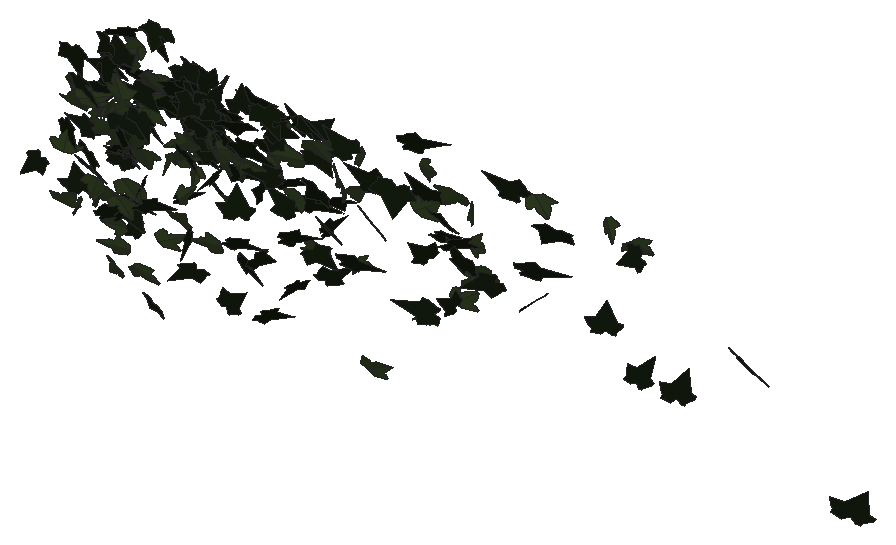
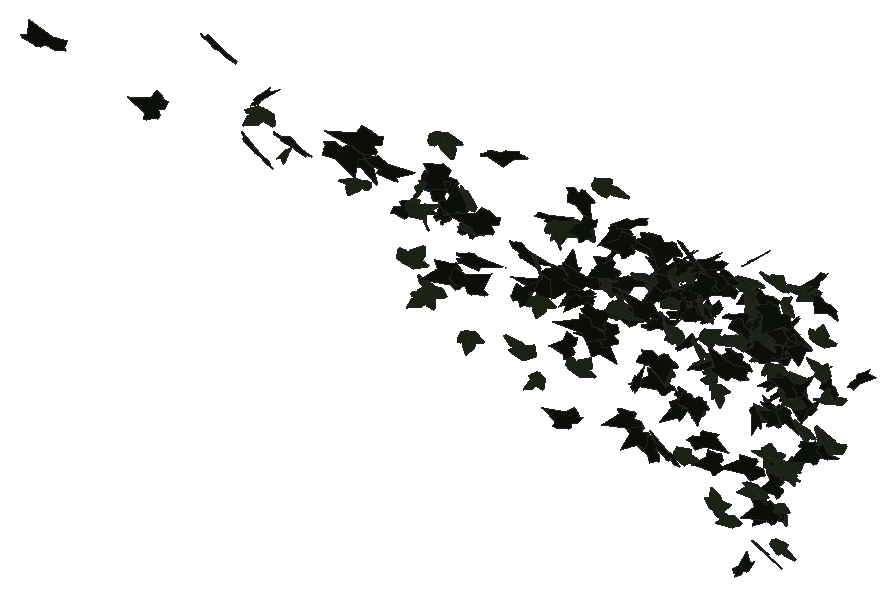
# SketchUp Ruby script. Lengths in millimetres.
U = 1.mm
M = Sketchup.active_model
def pt(a) = Geom::Point3d.new(a.map { |v| v * U })
def face(e, loops, mat)
  f = e.add_face(loops[0].map { |a| pt(a) })
  loops[1..].each { |l| e.add_face(l.map { |a| pt(a) }).erase! }
  f.material = f.back_material = mat if mat
  f
end
# faces: each face lists its corners as indices into pts; further lists are holes
def faces(e, pts, list, mat = nil) = list.each { |f| face(e, (f[0].is_a?(Array) ? f : [f]).map { |l| l.map { |i| pts[i] } }, mat) }
# xy, xz, yz: faces in a plane at the given z, y or x. An outline is a flat list of corners, or four numbers for a rectangle; further outlines are holes
def ring(l) = l.size == 4 ? [[l[0], l[1]], [l[2], l[1]], [l[2], l[3]], [l[0], l[3]]] : l.each_slice(2).to_a
def flat(e, list, mat, &to3) = list.each { |f| face(e, (f[0].is_a?(Array) ? f : [f]).map { |l| ring(l).map { |u, v| to3.(u, v) } }, mat) }
def xy(e, z, list, mat = nil) = flat(e, list, mat) { |x, y| [x, y, z] }
def xz(e, y, list, mat = nil) = flat(e, list, mat) { |x, z| [x, y, z] }
def yz(e, x, list, mat = nil) = flat(e, list, mat) { |y, z| [x, y, z] }
def lines(e, pts, list) = list.each { |a, b| e.add_line(pt(pts[a]), pt(pts[b])) }
# prism: a flat outline (further loops are holes) pulled along v
def prism(e, loops, v, mat = nil)
  f = face(e, loops, mat); d = Geom::Vector3d.new(v.map { |x| x * U })
  f.pushpull(f.normal.samedirection?(d) ? d.length : -d.length)
end
def box(e, o, s, mat = nil) = prism(e, [[o, [o[0] + s[0], o[1], o[2]], [o[0] + s[0], o[1] + s[1], o[2]], [o[0], o[1] + s[1], o[2]]]], [0, 0, s[2]], mat)
def at(x, y, z, deg = 0) = Geom::Transformation.translation(pt([x, y, z])) * Geom::Transformation.rotation(ORIGIN, Z_AXIS, deg.degrees)
def axes(o, x, y, z) = Geom::Transformation.new([*x, 0, *y, 0, *z, 0, *pt(o).to_a, 1])
def part(name) = M.definitions.add(name)
# library, detail: a bought-in or finely detailed component or shape, given as its bounding box
def library(name, o, s) = part(name).tap { |d| box(d.entities, o, s) }
def detail(e, o, s) = box(e.add_group.entities, o, s)
def put(e, d, t, mat = nil) = e.add_instance(d, t).tap { |i| i.material = mat if mat }
def group(e, t, mat = nil) = e.add_group.tap { |g| g.transformation = t; g.material = mat if mat }.entities
root = M.entities
M.materials.add("efeu1").color = [18, 25, 13]
M.materials.add("efeu2").color = [43, 57, 29]
c1 = part("ivyleaf_10")
p = [[0,12.8,-0.8],[-1.5,51.3,-10.9],[-4.9,51,-11.6],[-13.6,26.5,-7.3],[-13.2,15.9,-4.6],[-21.1,19.3,-7.2],
  [-29.5,16.3,-8.3],[-29.2,8.3,-6.2],[-19.7,-9.8,0.5],[-7.6,-13,4],[1,-12.2,5.8],[-0.4,51.1,-11.1],
  [-1.5,51.1,-10.9],[1,-12.4,5.9],[16.9,-12.4,3.5],[35.1,9.1,-5.1],[35,12.9,-6.1],[20.5,16.4,-4.9],
  [15.8,15,-3.8],[15.3,27.6,-7.1],[12.8,31.3,-7.8]]
faces(c1.entities,p,[[0,1,2,3,4,5,6,7,8,9,10],[11,12,0,13,14,15,16,17,18,19,20]],"efeu2")
c2 = part("ivyleaf_9")
p = [[39.1,54.8,31.7],[34.5,51.8,30.2],[-5.3,25.2,17.3],[-17.9,28.3,20.9],[-21.6,21.7,17],[-20.2,4.3,5.3],
  [-22.9,-0.3,2.5],[-17.1,-4,-0.6],[-2,-2.1,-1.2],[-0.7,-15.4,-10.1],[16.6,-22.3,-16.7],[21.1,-15.1,-12.5],
  [32.7,-10.7,-11],[46.1,-1.8,-6.6],[30.8,11.2,3.8]]
faces(c2.entities,p,[[0,1,2,3,4,5,6,7,8,9,10,11,12,13,14]],"efeu1")
put(root,c1,axes([5064.2,937.7,790.6],[0.67304,-0.23395,-0.96533],[-1.59231,0.48213,-0.42334],[1.0189,0.908,-0.02393]))
put(root,c1,axes([5001.8,756.4,1400.4],[-0.8248,0.04636,1.15791],[2.09058,-0.37742,0.42623],[0.70265,1.17734,0.09105]))
put(root,c2,axes([5054.6,918.4,1310.9],[-0.906,0.80347,-0.50065],[0.44749,-0.44248,-0.93368],[-1.74528,-0.53054,0.0205]))
put(root,c2,axes([5052.5,851.7,1350.8],[-0.03456,-0.01498,1.10733],[-1.36507,-0.84365,-0.02318],[1.60586,-0.71747,0.00413]))
put(root,c2,axes([5008.5,928.6,1425.8],[0.54035,-0.11605,-1.00857],[1.93217,0.03577,0.28167],[0.00611,-1.04716,0.12139]))
put(root,c2,axes([5023.9,778.4,1101],[1.95729,-0.44574,-0.06664],[-0.11819,0.02431,-1.12086],[0.84959,1.03029,-0.00239]))
put(root,c2,axes([5063,493,1250],[0.21616,-0.29781,-1.14485],[0.79529,-1.06587,0.31872],[-2.10625,-0.43302,0.00285]))
put(root,c2,axes([5081.5,705.2,1045.3],[-2.0987,-0.07093,0.2202],[0.4185,0.01182,1.105],[-0.13678,1.12443,0.00227]))
put(root,c1,axes([5057,640.6,1228.6],[1.69953,0.65213,-0.2656],[0.37803,0.17823,1.10545],[1.2857,-0.91444,0.02605]))
put(root,c2,axes([5045.2,662.6,1306.6],[-0.5613,0.05695,-1.17254],[2.19376,-0.21497,-0.30037],[-0.42323,-1.1898,-0.00186]))
put(root,c1,axes([5097.5,781.5,1320.9],[-0.42723,0.35407,1.05328],[-1.33204,0.78957,-0.41458],[-1.64262,-0.73237,0.06225]))
put(root,c1,axes([5069.2,624.9,1028.7],[-1.82637,-0.24048,0.45997],[0.87286,0.05985,0.98812],[-0.46254,1.06249,0.04845]))
put(root,c2,axes([5117.9,974.4,786.1],[-1.73472,0.56442,0.00038],[-0.00075,0.00009,-1.07208],[-1.0742,-0.91148,0.00014]))
put(root,c1,axes([5058.5,831,1298.2],[1.2924,-0.13297,-0.79694],[1.50662,-0.09878,0.69102],[-0.30766,-1.04235,0.03618]))
put(root,c2,axes([5078,657.6,1613.5],[-1.19341,-0.08927,-0.99726],[1.8737,0.15932,-0.6333],[0.34704,-1.16719,-0.01017]))
put(root,c1,axes([5100,775,1326.7],[0.10477,-1.00057,0.68235],[0.29766,-0.67147,-0.99722],[2.28566,0.13331,0.09859]))
put(root,c2,axes([5111.7,765.2,1278.7],[1.37307,0.31331,-0.76378],[-1.39675,-0.2211,-0.78392],[-0.71951,1.02712,0.06424]))
put(root,c2,axes([5105.9,820.3,1575.4],[-0.48565,-0.52996,0.88702],[-0.42571,-0.86368,-0.58036],[1.91991,-0.32557,0.09569]))
put(root,c2,axes([5130.5,687.2,1309.7],[-0.15478,-1.06398,-0.14432],[-0.02081,-0.14391,1.06708],[-2.04341,0.08206,0.00006]))
put(root,c1,axes([5140.4,794.6,1008.8],[-1.75315,0.04978,0.59176],[-1.12423,0.03547,-0.9225],[-0.11618,-1.09429,-0.00298]))
put(root,c1,axes([5132.4,618.4,1433.7],[-2.04621,0.21259,-0.09072],[-0.17772,-0.0047,1.09573],[0.40241,1.07895,0.02264]))
put(root,c2,axes([5116.7,781.6,1517],[0.72979,-0.5039,-1.08095],[-1.09473,0.91652,-0.6313],[1.98838,0.68955,0.04917]))
put(root,c2,axes([5092,932,909.9],[1.91135,0.05327,0.3186],[0.60672,0.00457,-1.00562],[-0.09927,1.0536,-0.01175]))
put(root,c2,axes([5103.9,712.7,1194.3],[0.13051,-0.86871,0.80221],[0.20025,-0.79588,-0.87086],[2.24152,0.12168,0.03109]))
put(root,c1,axes([5122.8,726.4,1012.3],[0.10372,-0.04255,-1.07115],[0.4224,1.04975,-0.03041],[1.99602,-0.21994,0.0621]))
put(root,c2,axes([5111.8,913.5,888.4],[-0.38965,-0.75246,-0.7988],[0.41389,0.76864,-0.7798],[2.04714,-0.29862,0.00562]))
put(root,c1,axes([5127.2,893.1,1101.8],[1.77653,0.55515,-0.12163],[0.16948,0.08812,1.08564],[1.06827,-0.9372,0.03003]))
put(root,c2,axes([5180.4,747.7,1527.9],[-0.73932,0.05518,-1.16046],[-2.21107,-0.01654,0.38811],[0.00344,1.22364,0.05758]))
put(root,c2,axes([5161.2,830.1,1519],[-2.17248,-0.10172,0.28438],[0.55274,-0.06455,1.14267],[-0.15776,1.17461,0.08742]))
put(root,c2,axes([5133.8,837.4,1630.3],[1.55878,0.87426,0.24465],[0.3207,0.17738,-1.19797],[-1.69779,0.83619,-0.00167]))
put(root,c1,axes([5152.2,602.8,1056.6],[0.49358,-1.13684,-0.16233],[-0.06031,0.15927,-1.16603],[2.18474,0.26123,0.00448]))
put(root,c2,axes([5161.3,722.3,1467.4],[1.32035,0.55576,-0.65751],[-0.96639,-0.41777,-0.88888],[-1.32317,0.8597,-0.0069]))
put(root,c1,axes([5185.8,723.3,1313.6],[-1.48603,-0.29671,0.77164],[-1.37717,-0.26803,-0.83527],[0.76094,-1.06454,-0.00477]))
put(root,c1,axes([5162.7,921.7,971.3],[1.56175,-0.62751,-0.26292],[-0.39992,0.15804,-1.03302],[1.23157,0.84707,-0.00204]))
put(root,c1,axes([5183.1,888.3,1555.9],[1.2385,-0.37421,-0.7487],[-1.25888,0.35123,-0.75045],[0.97616,0.92772,-0.01788]))
put(root,c1,axes([5155,684,1108.5],[1.9985,-0.54064,0.06378],[0.12765,-0.00903,-1.18086],[1.02818,1.05197,0.02264]))
put(root,c2,axes([5153.3,730.5,959],[0.20424,0.01435,1.07001],[1.70735,0.58507,-0.09782],[-1.11033,0.9023,0.0464]))
put(root,c2,axes([5167.5,798.2,924.4],[0.47641,0.37607,1.00371],[1.01539,0.85024,-0.45163],[-1.76927,0.58922,0.01108]))
put(root,c2,axes([5156.9,858.1,1469],[2.26962,-0.08387,-0.27225],[0.51652,-0.02173,1.19547],[-0.16481,-1.22302,-0.00257]))
put(root,c2,axes([5212.3,745.3,1430.6],[0.28079,-0.37544,1.02948],[-0.47608,0.9998,0.40047],[-2.03047,-0.28634,0.04847]))
put(root,c2,axes([5162.2,809.7,1197.8],[0.88049,-0.83971,0.54607],[0.55749,-0.46178,-0.95827],[1.823,0.54679,0.0293]))
put(root,c1,axes([5224.7,713.5,782.7],[-1.3865,0.38914,0.66141],[-1.12057,0.30146,-0.82588],[-0.9367,-0.93665,0.00898]))
put(root,c2,axes([5183.1,787.1,1326.2],[1.00325,-1.01866,0.01643],[0.01432,-0.01461,-1.14698],[1.93892,0.52719,-0.00003]))
put(root,c2,axes([5221.8,761,1240.2],[-0.60975,-0.56043,0.90184],[-0.88478,-0.77287,-0.64544],[1.8168,-0.56447,-0.01166]))
put(root,c2,axes([5213,748.8,1171.1],[-1.32421,0.67658,0.54301],[0.74321,-0.37732,0.9705],[1.47437,0.79787,-0.0015]))
put(root,c1,axes([5196.8,768.2,1005.9],[1.7398,0.19985,0.59739],[1.08677,0.18164,-0.93457],[-0.50621,1.07682,0.04678]))
put(root,c2,axes([5205.7,532.3,1596.1],[1.06998,-1.14469,-0.00344],[-0.00202,0.00331,-1.2753],[2.17858,0.5622,0.0005]))
put(root,c1,axes([5278.6,685.5,888.5],[0.01372,0.0139,1.08365],[-1.86185,-0.46623,0.01249],[0.88755,-0.97825,0.00945]))
put(root,c2,axes([5246.3,929.9,1627.8],[-1.21428,-0.87666,-0.02225],[0.0246,0.01811,-1.08425],[1.66881,-0.63815,-0.0002]))
put(root,c2,axes([5220.4,927.8,1594.9],[-0.4898,0.01277,-1.04929],[1.99688,-0.01471,-0.25752],[-0.03298,-1.08029,-0.0089]))
put(root,c1,axes([5269.3,717.8,1430.6],[1.30739,-0.61217,-0.63555],[-0.92869,0.40754,-0.91998],[1.3993,0.84245,-0.01677]))
put(root,c1,axes([5255.3,773.7,1553.5],[1.19116,-0.96913,0.5274],[-0.53739,0.44547,1.15365],[-2.02995,-0.68661,0.00407]))
put(root,c1,axes([5267,699.2,1308.1],[-1.13795,-0.9866,-0.20442],[0.22553,0.1672,-1.15354],[1.90426,-0.60937,0.01446]))
put(root,c1,axes([5237.4,526.7,1535.6],[0.89648,0.08984,-1.13989],[1.98945,0.46578,0.46867],[0.88192,-1.14205,0.10147]))
put(root,c2,axes([5250.3,829.5,988.4],[0.23583,0.43926,-1.00569],[0.47277,0.97459,0.45628],[2.03443,-0.2774,0.01055]))
put(root,c2,axes([5266.6,865.7,589],[1.21104,-0.642,-0.57517],[0.76326,-0.41233,0.9039],[-1.45212,-0.75214,-0.00458]))
put(root,c1,axes([5266,749.5,1384.8],[0.91172,0.46185,-0.89118],[1.22397,0.61694,0.66542],[1.46673,-0.80192,-0.00133]))
put(root,c2,axes([5283.3,805.8,1455.6],[0.45462,-0.51465,-1.0461],[1.05781,-0.88839,0.56399],[-1.95045,-0.60177,0.06204]))
put(root,c1,axes([5263.3,931.4,806.5],[1.31726,-0.04297,-0.81937],[1.56122,0.01368,0.69221],[-0.03286,-1.07249,0.04165]))
put(root,c1,axes([5298.1,598.8,1501.6],[0.50739,-0.99216,0.69498],[0.30977,-0.67582,-1.02724],[2.28454,0.312,-0.01506]))
put(root,c1,axes([5267.6,709.7,1124.4],[1.63569,0.05689,0.79181],[1.48973,0.13373,-0.85922],[-0.25177,1.16091,0.06018]))
put(root,c1,axes([5309.8,859.8,1485.3],[1.75949,0.48477,-0.38729],[-0.64796,-0.18468,-1.04387],[-0.98726,0.98517,-0.00511]))
put(root,c1,axes([5299.7,972.6,876.2],[-1.89439,0.16535,0.41323],[0.7465,-0.15257,1.00585],[0.40035,1.06688,0.0798]))
put(root,c2,axes([5326.2,721.5,1126.8],[-0.27138,0.12416,-1.22895],[-1.6277,0.88268,0.18841],[1.69618,0.86691,-0.01583]))
put(root,c1,axes([5275.4,770.5,1457.4],[0.62981,0.06052,-1.1124],[2.07001,0.23357,0.33627],[0.45883,-1.13683,0.00987]))
put(root,c2,axes([5280,866.3,1409.3],[-0.02432,0.0045,-1.1103],[1.94482,0.43433,-0.01],[0.82648,-1.02191,-0.00914]))
put(root,c2,axes([5293.9,668.2,1416.7],[-0.45715,-0.7174,-0.98343],[1.00062,0.84293,-0.74333],[2.08951,-0.56061,0.14081]))
put(root,c2,axes([5327.4,693.2,1331.7],[-0.86682,-0.7442,0.79182],[-0.69155,-0.70483,-0.87145],[1.94906,-0.58106,0.04295]))
put(root,c2,axes([5302.6,888.1,1354],[-0.92723,0.00001,1.14439],[1.86586,-0.64159,0.41738],[1.1235,1.06553,0.2513]))
put(root,c2,axes([5305.6,611,1324.6],[2.07086,0.26212,0.32005],[0.59143,0.0766,-1.11922],[-0.51973,1.1316,0.00162]))
put(root,c1,axes([5347.5,587.9,1564.7],[2.0483,-0.08575,0.44382],[-0.8361,0.07148,1.07913],[-0.20259,-1.16196,0.03363]))
put(root,c1,axes([5346.6,737.3,1573.4],[0.14783,-0.94291,0.60554],[0.18512,-0.59903,-0.94525],[2.12469,0.1178,0.04023]))
put(root,c1,axes([5323.8,711.2,810.7],[-1.24159,0.11669,-0.86899],[1.62988,-0.1475,-0.66272],[-0.35789,-1.07656,-0.00339]))
put(root,c2,axes([5340.9,915,1004.8],[0.66207,0.35599,0.95871],[1.35601,0.64209,-0.49695],[-1.39626,0.79238,-0.02802]))
put(root,c2,axes([5343.7,664.6,1554.9],[-0.6362,-0.44901,-1.13368],[1.50584,0.81456,-0.55592],[1.76578,-0.85642,0.06562]))
put(root,c2,axes([5345.1,582.9,1408.3],[0.24415,-0.08477,-1.23247],[2.26263,-0.3284,0.14633],[-0.63921,-1.19482,0.04722]))
put(root,c2,axes([5354,677.8,1454.4],[1.34868,-1.15375,-0.04659],[-0.02908,0.04529,-1.35395],[2.1974,0.70872,0.01068]))
put(root,c1,axes([5401.3,665,1473.9],[-0.03939,-1.07947,0.24208],[-0.02383,-0.24187,-1.07964],[2.10533,-0.02294,-0.00769]))
put(root,c1,axes([5402,840.1,1239],[-0.3553,-1.12325,-0.10035],[0.04219,0.09804,-1.13865],[2.14588,-0.18791,0.00577]))
put(root,c1,axes([5379.4,698,1587],[-0.61611,0.31033,-1.05872],[1.55034,-0.67688,-0.44749],[-1.41609,-0.87608,-0.02929]))
put(root,c1,axes([5412,572.4,1379.2],[-0.54332,-1.16466,-0.34594],[-0.15871,-0.33574,1.19914],[-2.30684,0.29741,-0.00102]))
put(root,c2,axes([5447,911.9,1216.2],[1.34732,0.21976,-0.8054],[-1.5276,-0.11126,-0.73587],[-0.43699,1.06651,0.08919]))
put(root,c1,axes([5447.4,875.8,1167.9],[0.26883,0.94566,-0.59477],[-0.21192,-0.5846,-0.95594],[-2.11557,0.17872,0.02018]))
put(root,c1,axes([5454.1,571.9,1373.5],[-2.17132,-0.33532,-0.23766],[0.4487,0.04044,-1.18883],[0.64072,-1.16467,0.02715]))
put(root,c2,axes([5478.9,855.5,1305.6],[-1.22545,-0.92695,0.25572],[0.27658,0.21041,1.12864],[-1.80905,0.66008,-0.00067]))
put(root,c1,axes([5455.8,720.6,1280.7],[0.22851,-0.39198,1.14556],[0.84926,-1.05582,-0.40804],[2.14213,0.4604,0.03957]))
put(root,c1,axes([5475.9,582.9,1530.2],[2.08777,0.24304,-0.16363],[-0.30359,-0.03646,-1.12358],[-0.46773,1.10852,-0.00108]))
put(root,c2,axes([5450,822.6,1618.8],[1.73634,-0.61368,0.33504],[0.55576,-0.16602,-1.09925],[1.20908,0.95761,0.02413]))
put(root,c1,axes([5524.2,739.7,1365.2],[-0.52299,-0.36508,1.04422],[-1.22038,-0.82417,-0.45689],[1.71552,-0.69759,-0.00668]))
put(root,c1,axes([5484.4,761.9,1270.5],[0.14668,-0.32794,1.07701],[0.49649,1.05535,0.30268],[-2.08437,0.22831,0.14789]))
put(root,c2,axes([5455,703.8,1572.8],[1.43973,0.33779,-0.92743],[1.46305,0.53128,0.82054],[1.17827,-1.07244,0.11438]))
put(root,c2,axes([5501,499.9,1573.1],[0.1418,-1.25549,0.12259],[0.03188,-0.12181,-1.25766],[2.4006,0.07578,0.00946]))
put(root,c1,axes([5515.3,805.4,1356],[1.68269,-0.70101,0.1802],[0.27684,-0.10659,-1.1283],[1.34944,0.896,0.00677]))
put(root,c1,axes([5563.1,837.9,931.1],[-0.4673,-0.01347,1.07701],[-2.01327,-0.20495,-0.24373],[0.38593,-1.08547,0.03266]))
put(root,c2,axes([5547.4,821.2,1551.3],[-0.25721,-0.10869,1.14619],[-1.65067,-0.74937,-0.17332],[1.44108,-0.87776,0.00605]))
put(root,c2,axes([5545.7,863.6,1185.7],[-1.15837,0.75542,-0.5157],[0.54571,-0.43064,-0.96922],[-1.65303,-0.67153,0.04141]))
put(root,c2,axes([5506.3,732.1,1657.7],[0.111,-0.64691,-0.92869],[0.32809,0.92415,-0.63292],[2.12889,-0.10869,0.14596]))
put(root,c1,axes([5532.2,690.8,1176.1],[0.14713,0.27266,-1.16452],[0.70735,1.1037,0.28309],[2.16357,-0.37938,-0.01336]))
put(root,c1,axes([5556.4,752.4,1509.8],[0.43537,-1.14299,-0.23813],[-0.06684,0.23581,-1.1656],[2.22104,0.23115,0.0116]))
put(root,c2,axes([5513.5,715.4,1605.3],[-0.35556,-0.06636,-1.28296],[2.34568,0.35651,-0.19791],[0.68981,-1.24651,0.01169]))
put(root,c2,axes([5532.3,874.5,1137.2],[1.79487,-0.57897,-0.34694],[-0.52648,0.21221,-1.10608],[1.17174,0.98221,0.03446]))
put(root,c2,axes([5567.1,817.1,1517.9],[0.44663,-0.25278,-1.10903],[-1.43301,0.81426,-0.34492],[1.62265,0.78867,0.00065]))
put(root,c1,axes([5567.9,686.6,1557.9],[-1.98959,-0.23981,-0.03283],[-0.04933,-0.03381,1.0722],[-0.45801,1.04536,0.02715]))
put(root,c2,axes([5583.4,711.6,1581.5],[-0.7729,-0.51323,1.09008],[-1.36167,-0.82283,-0.65395],[1.84501,-0.82227,-0.02599]))
put(root,c1,axes([5589.6,673.7,1413.3],[0.22644,-0.07677,-1.11055],[-0.9605,0.99178,-0.12263],[1.8884,0.51366,0.07079]))
put(root,c2,axes([5597.8,683.4,916.3],[0.03311,0.18419,-1.07806],[-0.3668,-1.06081,-0.18436],[-2.04893,0.19289,0.01558]))
put(root,c2,axes([5596.3,771.2,1314.7],[-1.06128,-0.72017,0.76162],[0.8741,0.6076,0.91079],[-1.79323,0.72239,-0.00679]))
put(root,c2,axes([5565.3,723.4,1437.8],[-0.73581,0.62953,0.98563],[1.00231,-0.83317,0.73873],[1.98738,0.65328,-0.00764]))
put(root,c2,axes([5629.5,715.6,1635.4],[-0.21142,0.57185,1.2489],[-0.76364,1.18482,-0.5782],[-2.50022,-0.41024,0.07099]))
put(root,c1,axes([5585.1,885.2,1424.6],[0.51172,-0.69444,-0.82511],[0.58932,-0.76485,0.74462],[-1.96607,-0.41,0.00844]))
put(root,c2,axes([5574.5,646.9,1388.9],[0.7121,-1.0394,0.54489],[0.34295,-0.51425,-1.10469],[2.20705,0.41527,-0.00415]))
put(root,c2,axes([5607.1,652.9,1588.7],[-0.76536,-0.86547,0.79158],[-0.56985,-0.73333,-0.9539],[2.15826,-0.50053,0.02885]))
put(root,c2,axes([5637.2,737.6,1398.5],[-2.06879,-0.50646,0.39007],[0.66761,0.17072,1.19918],[-1.01711,1.14219,-0.00628]))
put(root,c1,axes([5613.2,828.1,1603.5],[0.61121,-0.86475,0.72869],[0.53199,-0.6733,-0.9222],[2.08542,0.42521,0.02168]))
put(root,c2,axes([5619.2,751,1520.7],[-1.06736,-1.10055,-0.27464],[0.24642,0.24226,-1.23519],[2.14468,-0.57555,0.00524]))
put(root,c1,axes([5620.4,701.5,1558.2],[0.14197,-0.00351,-1.25714],[0.9578,1.15412,0.02664],[2.19252,-0.50395,0.06977]))
put(root,c1,axes([5617.4,717.6,1434.4],[-0.1702,0.09935,-1.22983],[0.90022,-1.13609,-0.12617],[-2.16883,-0.47935,0.04414]))
put(root,c2,axes([5632.1,701.6,1564.9],[-0.88853,-0.24231,1.14678],[1.86288,0.59845,0.52493],[-1.22713,1.08393,-0.03346]))
put(root,c1,axes([5630.1,767.5,1340.8],[-1.29798,0.68808,-0.743],[1.03681,-0.50584,-0.96849],[-1.62468,-0.87253,-0.02446]))
put(root,c2,axes([5668.3,832.1,1270.3],[1.31353,0.64815,-0.68048],[-0.94884,-0.46316,-0.9468],[-1.51613,0.85139,0.00298]))
put(root,c2,axes([5669.9,844.3,1503.1],[-1.0882,-0.56786,0.81892],[1.19247,0.52933,0.80452],[-1.47485,0.84697,0.04626]))
put(root,c2,axes([5638.1,925.4,1487],[0.154,-0.04723,1.21431],[1.58741,-0.88293,-0.08992],[1.68204,0.83758,-0.02632]))
put(root,c2,axes([5649.9,759.5,1523.3],[2.16882,0.07045,0.1905],[0.3603,0.02482,-1.14167],[-0.14001,1.15511,0.01291]))
put(root,c2,axes([5687,694.6,1510.7],[0.63807,-1.14336,-0.47479],[0.26818,-0.45346,1.19148],[-2.34089,-0.3636,0.00708]))
put(root,c2,axes([5689.7,674.5,1575.3],[-0.58211,-0.52476,0.89834],[-0.70827,-0.81922,-0.60525],[1.84904,-0.47901,0.05098]))
put(root,c1,axes([5707.8,753.9,1179.3],[-1.83957,0.42032,0.4684],[-0.82653,0.17584,-1.05395],[-0.86688,-1.05959,0.01091]))
put(root,c2,axes([5726.9,671.4,1531],[-0.49864,-0.95181,0.45422],[0.25492,0.43421,0.98713],[-1.99093,0.29398,0.01263]))
put(root,c2,axes([5675.4,844.3,911],[0.32303,0.00062,-1.15833],[2.18858,-0.14064,0.16843],[-0.26467,-1.16222,-0.021]))
put(root,c2,axes([5718.9,895.6,1164.5],[0.1166,0.09611,1.11467],[-0.97549,-0.98989,0.11352],[1.89271,-0.5161,-0.01016]))
put(root,c2,axes([5719.4,710.5,804.5],[-0.70555,0.74077,0.89729],[0.76674,-0.80177,0.82835],[2.07751,0.54748,-0.00098]))
put(root,c1,axes([5786.2,923.7,1462.5],[0.44451,0.08458,-1.10888],[-2.09994,0.15928,-0.22025],[0.26461,1.12196,0.11487]))
put(root,c2,axes([5742.9,832.5,945.1],[0.0021,0.12319,-1.16749],[-0.72273,1.10476,0.11621],[2.11418,0.37754,0.04088]))
put(root,c1,axes([5706.3,705.2,1420.8],[0.62918,-0.1268,-1.21528],[2.24376,-0.29772,0.35177],[-0.61106,-1.22375,0.04034]))
put(root,c2,axes([5742.2,659.4,1482.3],[0.52353,-0.4292,1.06823],[1.29853,-0.82385,-0.5067],[1.76476,0.73352,0.05594]))
put(root,c2,axes([5756.5,683.5,1076.8],[1.55973,0.28047,0.73328],[1.32886,0.22428,-0.86613],[-0.68317,1.07659,-0.01059]))
put(root,c2,axes([5802.9,633.5,1584.8],[1.56052,0.85897,-0.30443],[-0.44201,-0.19904,-1.18712],[-1.67716,0.85169,0.0296]))
put(root,c2,axes([5804.3,393.2,1251.5],[-1.17962,0.41507,-1.02408],[1.61766,-0.57121,-0.74595],[-1.34383,-1.05196,0.00099]))
put(root,c2,axes([5780.6,847.1,1416.1],[0.23223,0.11892,-1.14603],[1.01972,1.0144,0.16231],[1.94132,-0.54706,0.05184]))
put(root,c2,axes([5848.9,970.7,1420.6],[0.41746,-0.38978,1.09812],[-1.02663,0.9565,0.44726],[-1.96575,-0.58232,-0.00038]))
put(root,c2,axes([5833.1,625.2,1243.2],[-1.66564,-0.54852,0.80717],[1.28793,0.44009,1.03281],[-1.33826,1.10624,-0.01065]))
put(root,c1,axes([5833.3,646.4,1397],[-0.00174,-0.07634,-1.22885],[0.35799,1.21441,-0.07558],[2.31574,-0.18779,0.01076]))
put(root,c1,axes([5810.1,658.4,1429],[-0.27381,-0.1178,1.17235],[2.21161,0.18101,0.16079],[-0.37061,1.16719,0.09339]))
put(root,c1,axes([5849.3,794.2,1388.9],[1.11017,-0.32814,0.96519],[1.6224,-0.45286,-0.66915],[1.06405,1.03285,0.01325]))
put(root,c2,axes([5859.5,600.5,1536.3],[0.27352,0.09682,-1.25133],[2.08263,0.60712,0.17265],[1.16973,-1.10358,-0.0148]))
put(root,c2,axes([5888.9,713.3,1577.1],[0.53564,0.27325,1.10202],[1.598,0.71418,-0.39151],[-1.45459,0.88522,-0.0243]))
put(root,c2,axes([5946.9,690.5,1407.5],[-0.63905,-0.64961,-0.93352],[-0.64713,-0.87149,0.72875],[-2.06551,0.47402,0.0605]))
put(root,c2,axes([5910.2,679.2,1654.8],[-0.27322,-1.13895,-0.59227],[0.15696,0.58655,-1.14794],[2.43817,-0.16539,0.00753]))
put(root,c2,axes([5919.6,658.2,862.4],[0.01455,0.49498,-1.03911],[0.11184,1.03761,0.4947],[2.18769,-0.05634,-0.01838]))
put(root,c2,axes([5940.1,680.9,1560.8],[0.68825,-0.65673,-1.02545],[-0.82663,0.92979,-0.74864],[2.16513,0.56375,0.04015]))
put(root,c2,axes([5954.7,673.2,1598.5],[0.23372,-0.0497,-1.1794],[-0.5224,1.15206,-0.07713],[2.18505,0.28075,0.10771]))
put(root,c2,axes([5943.7,891.4,1487.1],[-1.04163,0.13761,0.99211],[1.83055,-0.24325,0.56434],[0.53189,1.10664,0.00068]))
put(root,c2,axes([5971,880,1419.5],[-0.20407,-0.83999,-0.77111],[0.12491,0.76868,-0.84647],[2.16655,-0.12344,-0.02383]))
put(root,c2,axes([5974,802.3,1267.3],[0.64748,0.381,-1.06977],[1.29317,0.82649,0.51044],[1.73169,-0.75965,0.01881]))
put(root,c2,axes([6056.1,643.6,1328.7],[-1.93768,-0.10373,-0.49978],[-0.94594,-0.05239,1.02339],[-0.22116,1.13296,0.00156]))
put(root,c1,axes([6043.1,811.8,1084.6],[-1.91748,0.02707,-0.55302],[-1.05325,-0.01347,1.00756],[0.03281,1.14922,0.02484]))
put(root,c2,axes([5995.3,682.9,1177.7],[1.04867,0.29744,1.04548],[1.78145,0.46604,-0.62591],[-1.05169,1.08602,-0.01774]))
put(root,c2,axes([6005.1,897.4,927.5],[-0.19446,-0.07352,1.13697],[2.03223,0.39198,0.12131],[-0.75632,1.07215,0.03361]))
put(root,c2,axes([6021.1,647.4,1418.1],[1.12705,0.6415,0.72569],[0.95241,0.52561,-0.873],[-1.57829,0.77526,-0.0086]))
put(root,c1,axes([6066.7,657.3,1374.5],[1.64273,-0.66882,-0.56296],[-0.80835,0.37065,-1.09155],[1.45423,0.96154,0.02919]))
put(root,c2,axes([6030.7,760.1,1612.9],[1.55953,-0.9613,0.3054],[0.38056,-0.23086,-1.26315],[1.88155,0.84347,0.00234]))
put(root,c2,axes([6058.4,822.9,1168.2],[0.21307,0.17922,1.19397],[1.45707,0.91665,-0.20938],[-1.77676,0.77321,-0.02852]))
put(root,c2,axes([6115.2,606,1076.2],[-0.44703,0.76108,-0.84981],[0.37282,-0.82784,-0.79555],[-2.13891,-0.30336,0.03894]))
put(root,c1,axes([6100,706.8,1574.5],[-1.92747,0.0091,-0.62295],[1.18565,0.00121,-1.01278],[-0.01355,-1.189,-0.0058]))
put(root,c1,axes([6177.3,513.9,1629.8],[-0.44335,-0.03972,1.18082],[-2.01107,-0.5314,-0.22633],[1.00589,-1.07992,0.06795]))
put(root,c1,axes([6155.2,878.8,1343.3],[-1.21336,-0.94943,-0.20202],[0.23885,0.15905,-1.14352],[1.83191,-0.64959,0.01529]))
put(root,c1,axes([6165.7,762,1582.7],[-1.39225,-0.96042,0.00524],[-0.00334,-0.00525,-1.20729],[1.8279,-0.73153,0.00179]))
put(root,c1,axes([6152.6,887.4,1044.7],[-0.45177,-0.55953,-0.98755],[0.81979,0.88903,-0.60725],[1.99862,-0.49114,0.02586]))
put(root,c2,axes([6161,726,1369.8],[1.59268,0.85483,-0.00621],[-0.01717,0.00015,-1.19625],[-1.62687,0.83687,0.00655]))
put(root,c1,axes([6180.3,867.9,1491.4],[0.87902,-0.99398,-0.39492],[-0.31251,0.35918,-1.09604],[2.01145,0.49018,0.0023]))
put(root,c2,axes([6229.6,740.7,1578],[-1.98163,-0.48177,-0.21139],[-0.36398,-0.09006,1.14727],[-0.93279,1.05863,0.0014]))
put(root,c1,axes([6226,681,1491.5],[-0.04317,0.26617,-1.21831],[-0.70116,1.1627,0.26088],[2.26745,0.36461,0.05747]))
put(root,c2,axes([6193.8,592.8,1238.6],[0.10869,-0.50346,-1.05805],[-0.03083,1.05886,-0.50472],[2.22981,0.03918,0.04459]))
put(root,c2,axes([6226,630.5,1315.1],[1.58592,-0.79717,-0.25299],[0.35241,-0.17242,1.15319],[-1.55225,-0.85361,0.00333]))
put(root,c2,axes([6298.2,795,1444.5],[-0.59814,0.32401,1.14201],[-1.52878,0.81177,-0.45137],[-1.66346,-0.86255,0.00419]))
put(root,c2,axes([6281.7,497.9,1549.9],[1.06865,0.09489,-1.07433],[-2.03715,-0.09938,-0.56822],[-0.25151,1.20813,0.03764]))
put(root,c1,axes([6268.9,659.6,1463.7],[-0.94503,0.75485,0.81094],[0.87389,-0.66853,0.90345],[1.91892,0.6762,-0.01206]))
put(root,c2,axes([6297.4,805.5,1267.2],[0.76376,-1.0213,0.56979],[-0.40543,0.52849,1.09731],[-2.18855,-0.45432,-0.00443]))
put(root,c2,axes([6307.6,622.5,1222],[1.10807,-0.08392,1.00036],[1.8786,-0.16281,-0.58814],[0.34805,1.14594,-0.0103]))
put(root,c2,axes([6402.6,968.5,1354.7],[0.98938,-0.27528,1.09128],[-1.84583,0.50031,0.58821],[-1.08675,-1.10038,-0.00556]))
put(root,c2,axes([6355.4,905,1581.5],[0.78734,0.10407,1.21451],[2.28424,0.18934,-0.42505],[-0.4054,1.26899,-0.03618]))
put(root,c1,axes([6468.1,564.3,886.1],[-1.525,-0.13054,0.8762],[1.64554,0.14198,0.81185],[-0.36707,1.17882,-0.00075]))
put(root,c1,axes([6498.4,816.2,1578.5],[0.3572,-0.2549,-1.14409],[1.21493,-0.94953,0.31628],[-1.87097,-0.66525,-0.01305]))
put(root,c1,axes([6538.5,787.6,1030.3],[-0.91043,-1.10896,-0.32044],[0.24036,0.29451,-1.20774],[2.18374,-0.49476,-0.00066]))
put(root,c1,axes([6520.6,766.7,1441.7],[1.75464,-0.24677,-0.78772],[1.45492,-0.19032,0.95434],[-0.59276,-1.19761,0.01065]))
put(root,c2,axes([6534.5,857.5,1301.8],[2.01552,0.1704,0.5293],[0.99386,0.08642,-1.07263],[-0.36359,1.18077,0.00212]))
put(root,c2,axes([6576.8,559.1,1635.6],[-1.44612,-1.0919,-0.33191],[0.34695,0.2775,-1.33023],[2.14409,-0.78135,-0.00861]))
put(root,c2,axes([6640.3,653.1,1345.1],[0.46654,0.29945,1.19139],[-1.82949,-0.70966,0.37616],[1.4557,-0.98786,0.09092]))
put(root,c2,axes([6642.3,723.3,1458.8],[2.00289,-0.65689,-0.06147],[0.15093,0.01106,1.2395],[-1.24655,-1.05412,0.05131]))
put(root,c2,axes([6717.3,583.4,1182],[-1.12657,-0.48871,-0.9175],[-1.25303,-0.64083,0.7661],[-1.53107,0.88405,0.04813]))
put(root,c1,axes([6667.5,862.7,1173.5],[-1.07335,-0.56407,-0.90508],[1.18049,0.65937,-0.79744],[1.65109,-0.83813,-0.01823]))
put(root,c1,axes([6678.3,848.2,1461.9],[0.36675,-0.31179,1.15088],[1.35206,-0.90628,-0.36448],[1.82256,0.73506,0.0388]))
put(root,c1,axes([6689,773.8,1138.7],[1.79967,-0.12598,-0.74227],[1.39984,-0.0999,0.95396],[-0.30599,-1.19798,-0.00149]))
put(root,c1,axes([6783.7,625,1653.5],[-2.11689,-0.23607,0.54624],[-1.02077,-0.10386,-1.13702],[0.49057,-1.23481,-0.00879]))
put(root,c1,axes([6798.8,784.6,1233.5],[-1.55755,-0.62266,-0.7283],[-1.08307,-0.45472,1.02823],[-1.46718,0.99669,0.01412]))
put(root,c2,axes([6793.2,587.1,1478.3],[1.5286,0.7267,0.76336],[1.0929,0.50305,-1.08309],[-1.68199,0.98729,-0.01001]))
put(root,c2,axes([6856.3,593.3,1403.6],[0.65008,-0.47745,1.19621],[-1.04469,1.06558,0.58205],[-2.21751,-0.64197,0.07647]))
put(root,c1,axes([6836.3,668.6,1457.4],[-0.27947,0.84859,0.92094],[-0.39315,0.89813,-0.86051],[-2.3507,-0.2511,0.03443]))
put(root,c2,axes([6882.8,844,1591.9],[-0.24259,0.05752,1.21771],[-1.99697,0.61812,-0.13903],[-1.18115,-1.05688,-0.01504]))
put(root,c2,axes([6853.2,538.6,1275.8],[0.15915,0.08942,1.2258],[-1.48822,-0.94402,0.12221],[1.80465,-0.78638,-0.00732]))
put(root,c1,axes([6876,664.3,1353.3],[-0.58605,-0.25474,-1.15462],[-1.76449,-0.68848,0.39915],[-1.39662,0.97672,-0.01978]))
put(root,c2,axes([6928.8,657.5,1345.4],[-0.26638,-0.28727,-1.18433],[-0.26132,-1.18081,0.30264],[-2.30461,0.1671,0.10258]))
put(root,c1,axes([6916.9,911.8,1554.4],[1.45061,0.8917,0.39726],[0.51032,0.29338,-1.17299],[-1.78642,0.80789,-0.0125]))
put(root,c2,axes([7105.2,770.6,1560.2],[1.24862,0.56023,-0.89357],[-1.27005,-0.59441,-0.86261],[-1.55435,0.93572,-0.01297]))
put(root,c2,axes([7196.8,558.7,1411.4],[-0.61423,1.1635,-0.38276],[0.19567,-0.36869,-1.20743],[-2.32289,-0.33872,-0.0005]))
put(root,c2,axes([7126.2,588.8,1488.9],[1.09741,-0.0393,1.19422],[2.27373,0.04229,-0.57545],[-0.04001,1.32547,0.05377]))
put(root,c1,axes([7231.8,909.9,1571.3],[0.02446,1.26224,-0.10688],[-0.02012,-0.10677,-1.26227],[-2.4108,0.0137,0.00945]))
put(root,c1,axes([7425.8,810.8,1606],[-1.37567,-0.60275,-0.85395],[1.25141,0.54488,-0.94116],[1.54639,-0.97714,0.00195]))
put(root,c2,axes([7466.1,602.5,1374],[-2.1475,0.5835,0.09378],[0.15863,-0.04298,1.2703],[1.11352,1.13144,-0.00011]))
put(root,c2,axes([7499.5,744.4,1604.2],[-0.62952,-0.54169,1.10762],[-1.16484,-0.92339,-0.63436],[2.03709,-0.69541,-0.02045]))
put(root,c2,axes([7643.6,554.8,1251.6],[-1.35832,1.09514,0.52343],[0.48688,-0.45785,1.30676],[2.25822,0.75745,0.0331]))
put(root,c2,axes([8015.3,308.5,1425.3],[-1.97716,0.95051,0.26711],[0.36465,-0.18629,1.40806],[1.84337,1.05635,0.00796]))
put(root,c2,axes([7968.7,709.1,1384.9],[1.20863,-0.91114,0.82224],[0.91672,-0.66649,-1.11055],[2.14838,0.79698,0.0113]))
put(root,c2,axes([8754.1,341,1205.7],[-1.81947,0.13412,0.99079],[1.83382,-0.24232,0.96253],[0.50792,1.35532,0.07405]))
